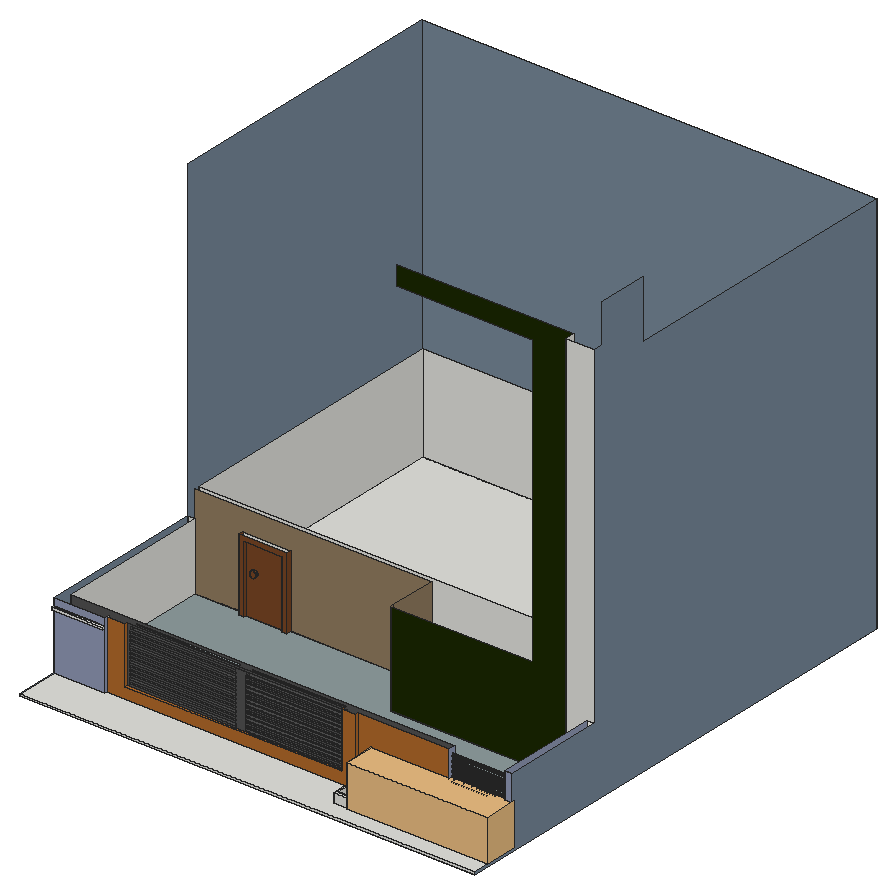
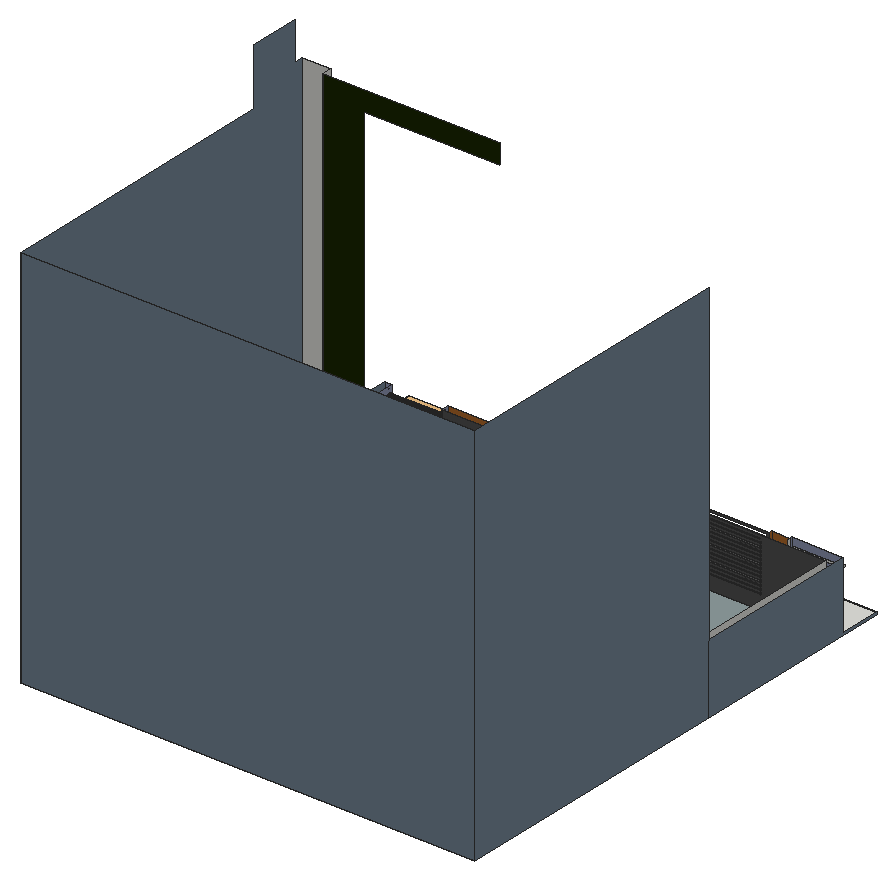
# SketchUp Ruby script. Lengths in inches.
U = 1.inch
M = Sketchup.active_model
def pt(a) = Geom::Point3d.new(a.map { |v| v * U })
def face(e, loops, mat)
  f = e.add_face(loops[0].map { |a| pt(a) })
  loops[1..].each { |l| e.add_face(l.map { |a| pt(a) }).erase! }
  f.material = f.back_material = mat if mat
  f
end
# faces: each face lists its corners as indices into pts; further lists are holes
def faces(e, pts, list, mat = nil) = list.each { |f| face(e, (f[0].is_a?(Array) ? f : [f]).map { |l| l.map { |i| pts[i] } }, mat) }
# xy, xz, yz: faces in a plane at the given z, y or x. An outline is a flat list of corners, or four numbers for a rectangle; further outlines are holes
def ring(l) = l.size == 4 ? [[l[0], l[1]], [l[2], l[1]], [l[2], l[3]], [l[0], l[3]]] : l.each_slice(2).to_a
def flat(e, list, mat, &to3) = list.each { |f| face(e, (f[0].is_a?(Array) ? f : [f]).map { |l| ring(l).map { |u, v| to3.(u, v) } }, mat) }
def xy(e, z, list, mat = nil) = flat(e, list, mat) { |x, y| [x, y, z] }
def xz(e, y, list, mat = nil) = flat(e, list, mat) { |x, z| [x, y, z] }
def yz(e, x, list, mat = nil) = flat(e, list, mat) { |y, z| [x, y, z] }
def lines(e, pts, list) = list.each { |a, b| e.add_line(pt(pts[a]), pt(pts[b])) }
# prism: a flat outline (further loops are holes) pulled along v
def prism(e, loops, v, mat = nil)
  f = face(e, loops, mat); d = Geom::Vector3d.new(v.map { |x| x * U })
  f.pushpull(f.normal.samedirection?(d) ? d.length : -d.length)
end
def box(e, o, s, mat = nil) = prism(e, [[o, [o[0] + s[0], o[1], o[2]], [o[0] + s[0], o[1] + s[1], o[2]], [o[0], o[1] + s[1], o[2]]]], [0, 0, s[2]], mat)
def at(x, y, z, deg = 0) = Geom::Transformation.translation(pt([x, y, z])) * Geom::Transformation.rotation(ORIGIN, Z_AXIS, deg.degrees)
def axes(o, x, y, z) = Geom::Transformation.new([*x, 0, *y, 0, *z, 0, *pt(o).to_a, 1])
def part(name) = M.definitions.add(name)
# library, detail: a bought-in or finely detailed component or shape, given as its bounding box
def library(name, o, s) = part(name).tap { |d| box(d.entities, o, s) }
def detail(e, o, s) = box(e.add_group.entities, o, s)
def put(e, d, t, mat = nil) = e.add_instance(d, t).tap { |i| i.material = mat if mat }
def group(e, t, mat = nil) = e.add_group.tap { |g| g.transformation = t; g.material = mat if mat }.entities
root = M.entities
M.materials.add("Niraj_Shirt").color = [144, 153, 181]
M.materials.add("[0035_Tan]").color = [145, 124, 96]
M.materials.add("[0060_GrassGreen]").color = [27, 40, 2]
M.materials.add("[0110_LightSlateGray]").color = [119, 136, 153]
M.materials.add("[0135_DarkGray]").color = [81, 81, 81]
M.materials.add("[0136_Charcoal]").color = [35, 35, 35]
M.materials.add("[Metal Panel]").color = [143, 157, 158]
M.materials.add("[Wood Bamboo]").color = [177, 105, 43]
M.materials.add("[Wood Veneer 01]").color = [120, 70, 37]
c1 = library("Potted flowering plants",[-0.05,-0.05,0],[59.02,14.54,22.0625])
xy(root,0,[[3.53,0,3.53,261.0625,307.22,261.0625,307.22,198.0625,534.65,198.0625,534.65,186.0625,569.78,186.0625,569.78,0],[534.65,186.0625,569.78,198.0625],[307.22,198.0625,450.59,261.0625],[450.59,198.0625,459.59,261.0625],[459.59,198.0625,569.78,261.0625],
  [[3.53,261.0625,569.78,625.1875],[12.53,267.0625,450.59,616.1875]],[12.53,267.0625,450.59,616.1875]])
xy(root,3,[[3.53,0,569.78,0,569.78,20.66,377.85,20.66,377.85,55.23,67.4,55.23,67.4,52.23,3.53,52.23],[381.12,23.93,566.51,58.23],[71.58,255.0625,77.58,261.0625],[125.58,255.0625,131.58,261.0625],[77.58,258.0625,125.58,261.0625]])
xy(root,3,[[12.53,67.23,560.78,67.23,560.78,186.0625,534.65,186.0625,534.65,198.0625,307.22,198.0625,307.22,261.0625,131.58,261.0625,131.58,255.0625,125.58,255.0625,125.58,258.0625,77.58,258.0625,77.58,255.0625,71.58,255.0625,71.58,261.0625,12.53,261.0625]],"[Metal Panel]")
xy(root,15,[[377.85,20.66,569.78,20.66,569.78,58.23,566.51,58.23,566.51,23.93,381.12,23.93,381.12,58.23,377.85,58.23]])
xy(root,17.19,[[90.07,55.23,224.96,58.23],[224.96,55.23,238.29,58.23],[238.29,55.23,359.85,58.23]],"[Wood Bamboo]")
xy(root,18.47,[[238.29,58.23,356.85,67.23]],"[0135_DarkGray]")
xy(root,19.75,[[93.07,58.23,224.96,67.23]],"[0135_DarkGray]")
xy(root,21.1875,[[238.29,58.23,356.85,67.23]],"[0135_DarkGray]")
xy(root,22.25,[[93.07,58.23,224.96,67.23]],"[0135_DarkGray]")
xy(root,22.66,[[238.29,58.23,356.85,67.23]],"[0135_DarkGray]")
xy(root,24.5,[[93.07,58.23,224.96,67.23]],"[0135_DarkGray]")
xy(root,25.375,[[238.29,58.23,356.85,67.23]],"[0135_DarkGray]")
xy(root,26.85,[[238.29,58.23,356.85,67.23]],"[0135_DarkGray]")
xy(root,27,[[93.07,58.23,224.96,67.23]],"[0135_DarkGray]")
xy(root,29.25,[[93.07,58.23,224.96,67.23]],"[0135_DarkGray]")
xy(root,29.5625,[[238.29,58.23,356.85,67.23]],"[0135_DarkGray]")
xy(root,31.03,[[238.29,58.23,356.85,67.23]],"[0135_DarkGray]")
xy(root,31.75,[[93.07,58.23,224.96,67.23]],"[0135_DarkGray]")
xy(root,33.75,[[238.29,58.23,356.85,67.23]],"[0135_DarkGray]")
xy(root,34,[[93.07,58.23,224.96,67.23]],"[0135_DarkGray]")
xy(root,35.22,[[238.29,58.23,356.85,67.23]],"[0135_DarkGray]")
xy(root,36.5,[[93.07,58.23,224.96,67.23]],"[0135_DarkGray]")
xy(root,37.9375,[[238.29,58.23,356.85,67.23]],"[0135_DarkGray]")
xy(root,38.75,[[93.07,58.23,224.96,67.23]],"[0135_DarkGray]")
xy(root,39.41,[[238.29,58.23,356.85,67.23]],"[0135_DarkGray]")
xy(root,41.25,[[93.07,58.23,224.96,67.23]],"[0135_DarkGray]")
xy(root,42.125,[[238.29,58.23,356.85,67.23]],"[0135_DarkGray]")
xy(root,43.5,[[93.07,58.23,224.96,67.23]],"[0135_DarkGray]")
xy(root,43.6,[[238.29,58.23,356.85,67.23]],"[0135_DarkGray]")
xy(root,45,[[491.3125,58.23,560.78,67.23]],"Niraj_Shirt")
xy(root,46,[[93.07,58.23,224.96,67.23]],"[0135_DarkGray]")
xy(root,46.3125,[[238.29,58.23,356.85,67.23]],"[0135_DarkGray]")
xy(root,47.78,[[238.29,58.23,356.85,67.23]],"[0135_DarkGray]")
xy(root,48.25,[[93.07,58.23,224.96,67.23]],"[0135_DarkGray]")
xy(root,50.5,[[238.29,58.23,356.85,67.23]],"[0135_DarkGray]")
xy(root,50.75,[[93.07,58.23,224.96,67.23]],"[0135_DarkGray]")
xy(root,51.97,[[238.29,58.23,356.85,67.23]],"[0135_DarkGray]")
xy(root,53,[[93.07,58.23,224.96,67.23]],"[0135_DarkGray]")
xy(root,54.6875,[[238.29,58.23,356.85,67.23]],"[0135_DarkGray]")
xy(root,55.5,[[93.07,58.23,224.96,67.23]],"[0135_DarkGray]")
xy(root,56.16,[[238.29,58.23,356.85,67.23]],"[0135_DarkGray]")
xy(root,57.75,[[93.07,58.23,224.96,67.23]],"[0135_DarkGray]")
xy(root,58.875,[[238.29,58.23,356.85,67.23]],"[0135_DarkGray]")
xy(root,60.25,[[93.07,58.23,224.96,67.23]],"[0135_DarkGray]")
xy(root,60.35,[[238.29,58.23,356.85,67.23]],"[0135_DarkGray]")
xy(root,62.5,[[93.07,58.23,224.96,67.23]],"[0135_DarkGray]")
xy(root,63.0625,[[238.29,58.23,356.85,67.23]],"[0135_DarkGray]")
xy(root,64.53,[[238.29,58.23,356.85,67.23]],"[0135_DarkGray]")
xy(root,65,[[93.07,58.23,224.96,67.23]],"[0135_DarkGray]")
xy(root,67.25,[[93.07,58.23,224.96,67.23],[238.29,58.23,356.85,67.23]],"[0135_DarkGray]")
xy(root,68.72,[[238.29,58.23,356.85,67.23]],"[0135_DarkGray]")
xy(root,69.75,[[93.07,58.23,224.96,67.23]],"[0135_DarkGray]")
xy(root,71.4375,[[238.29,58.23,356.85,67.23]],"[0135_DarkGray]")
xy(root,72,[[93.07,58.23,224.96,67.23]],"[0135_DarkGray]")
xy(root,72.91,[[238.29,58.23,356.85,67.23]],"[0135_DarkGray]")
xy(root,74.5,[[93.07,58.23,224.96,67.23]],"[0135_DarkGray]")
xy(root,74.66,[[3.53,49.23,67.4,52.23]])
xy(root,75.625,[[238.29,58.23,356.85,67.23]],"[0135_DarkGray]")
xy(root,76.75,[[93.07,58.23,224.96,67.23]],"[0135_DarkGray]")
xy(root,77.1,[[238.29,58.23,356.85,67.23]],"[0135_DarkGray]")
xy(root,77.67,[[3.53,49.23,67.4,52.23]])
xy(root,79.25,[[93.07,58.23,224.96,67.23]],"[0135_DarkGray]")
xy(root,79.8125,[[238.29,58.23,356.85,67.23]],"[0135_DarkGray]")
xz(root,0,[[3.53,0,569.78,3]])
xz(root,20.66,[[377.85,3,569.78,15]])
xz(root,23.93,[[381.12,3,566.51,15]])
xz(root,49.23,[[3.53,74.66,67.4,77.67]])
xz(root,52.23,[[3.53,74.66,67.4,77.67]])
xz(root,52.23,[[3.53,3,67.4,74.66],[3.53,77.67,67.4,87]],"Niraj_Shirt")
xz(root,55.23,[[67.4,3,377.85,3,377.85,87,359.85,87,359.85,17.19,90.07,17.19,90.07,87,67.4,87]],"[Wood Bamboo]")
xz(root,58.23,[[377.85,3,381.12,15]])
xz(root,58.23,[[491.09,3,566.51,3,566.51,15,569.78,15,569.78,87,560.78,87,560.78,45,491.3125,45,491.3125,87,491.09,87]],"Niraj_Shirt")
xz(root,58.23,[[90.07,17.19,224.96,17.19,224.96,19.75,93.07,19.75,93.07,84,356.85,84,356.85,18.47,238.29,18.47,238.29,17.19,359.85,17.19,359.85,87,90.07,87],[224.96,17.19,238.29,84],[238.29,21.1875,356.85,22.66],[93.07,22.25,224.96,24.5],[238.29,25.375,356.85,26.85],
  [93.07,27,224.96,29.25],[238.29,29.5625,356.85,31.03],[93.07,31.75,224.96,34],[238.29,33.75,356.85,35.22],[93.07,36.5,224.96,38.75],
  [238.29,37.9375,356.85,39.41],[93.07,41.25,224.96,43.5],[238.29,42.125,356.85,43.6],[93.07,46,224.96,48.25],[238.29,46.3125,356.85,47.78],
  [238.29,50.5,356.85,51.97],[93.07,50.75,224.96,53],[238.29,54.6875,356.85,56.16],[93.07,55.5,224.96,57.75],[238.29,58.875,356.85,60.35],
  [93.07,60.25,224.96,62.5],[238.29,63.0625,356.85,64.53],[93.07,65,224.96,67.25],[238.29,67.25,356.85,68.72],[93.07,69.75,224.96,72],
  [238.29,71.4375,356.85,72.91],[93.07,74.5,224.96,76.75],[238.29,75.625,356.85,77.1],[93.07,79.25,224.96,81.5],[238.29,79.8125,356.85,81.28]],"[0135_DarkGray]")
xz(root,58.23,[[381.12,3,491.09,3,491.09,87,377.85,87,377.85,15,381.12,15]],"[Wood Bamboo]")
xz(root,67.23,[[[12.53,3,12.53,87,491.3125,87,491.3125,45,560.78,45,560.78,3],[93.07,81.5,224.96,84],[93.07,76.75,224.96,79.25],[93.07,72,224.96,74.5],[93.07,67.25,224.96,69.75],[93.07,62.5,224.96,65],[93.07,57.75,224.96,60.25],[93.07,53,224.96,55.5],[93.07,48.25,224.96,50.75],[93.07,43.5,224.96,46],[93.07,38.75,224.96,41.25],[93.07,34,224.96,36.5],[93.07,29.25,224.96,31.75],[93.07,24.5,224.96,27],[93.07,19.75,224.96,22.25],[238.29,18.47,356.85,21.1875],[238.29,81.28,356.85,84],[238.29,77.1,356.85,79.8125],[238.29,72.91,356.85,75.625],[238.29,68.72,356.85,71.4375],[238.29,64.53,356.85,67.25],[238.29,60.35,356.85,63.0625],[238.29,56.16,356.85,58.875],[238.29,51.97,356.85,54.6875],[238.29,47.78,356.85,50.5],[238.29,43.6,356.85,46.3125],[238.29,39.41,356.85,42.125],[238.29,35.22,356.85,37.9375],[238.29,31.03,356.85,33.75],[238.29,26.85,356.85,29.5625],[238.29,22.66,356.85,25.375]]],"[0135_DarkGray]")
xz(root,186.0625,[[534.65,3,560.78,3,560.78,87,569.78,87,569.78,504.07,534.65,504.07]])
xz(root,198.0625,[[307.22,0,450.59,3],[450.59,0,534.65,3]])
xz(root,198.0625,[[307.22,3,534.65,3,534.65,504.07,314.59,504.07,314.59,480,483.9,480,483.9,120,307.22,120]],"[0060_GrassGreen]")
xz(root,255.0625,[[71.58,3,77.58,3,77.58,87,125.58,87,125.58,3,131.58,3,131.58,93,71.58,93],[88.84,49.68,89.86,49.82,90.8125,50.21,91.63,50.84,92.25,51.65,92.65,52.6,92.78,53.62,92.65,54.64,92.25,55.59,91.63,56.41,90.8125,57.03,89.86,57.42,88.84,57.56,87.83,57.42,86.875,57.03,86.0625,56.41,85.43,55.59,85.04,54.64,84.91,53.62,85.04,52.6,85.43,51.65,86.0625,50.84,86.875,50.21,87.83,49.82]],"[Wood Veneer 01]")
xz(root,258.0625,[[88.84,49.68,87.83,49.82,86.875,50.21,86.0625,50.84,85.43,51.65,85.04,52.6,84.91,53.62,85.04,54.64,85.43,55.59,86.0625,56.41,86.875,57.03,87.83,57.42,88.84,57.56,89.86,57.42,90.8125,57.03,91.63,56.41,92.25,55.59,92.65,54.64,92.78,53.62,92.65,52.6,92.25,51.65,91.63,50.84,90.8125,50.21,89.86,49.82]])
xz(root,258.0625,[[[77.58,3,125.58,87],[88.84,49.68,87.83,49.82,86.875,50.21,86.0625,50.84,85.43,51.65,85.04,52.6,84.91,53.62,85.04,54.64,85.43,55.59,86.0625,56.41,86.875,57.03,87.83,57.42,88.84,57.56,89.86,57.42,90.8125,57.03,91.63,56.41,92.25,55.59,92.65,54.64,92.78,53.62,92.65,52.6,92.25,51.65,91.63,50.84,90.8125,50.21,89.86,49.82]]],"[Wood Veneer 01]")
xz(root,261.0625,[[3.53,0,12.53,3],[12.53,0,71.58,3],[71.58,0,131.58,3],[131.58,0,307.22,3],[3.53,3,12.53,87]])
xz(root,261.0625,[[12.53,3,71.58,3,71.58,93,131.58,93,131.58,3,307.22,3,307.22,120,12.53,120]],"[0035_Tan]")
xz(root,267.0625,[[12.53,0,450.59,120]])
xz(root,616.1875,[[12.53,0,450.59,120]])
xz(root,625.1875,[[3.53,0,569.78,480]],"[0110_LightSlateGray]")
yz(root,3.53,[[49.23,74.66,52.23,77.67]])
yz(root,3.53,[[0,0,0,3,52.23,3,52.23,87,261.0625,87,261.0625,0],[261.0625,0,625.1875,480]],"[0110_LightSlateGray]")
yz(root,12.53,[[267.0625,0,616.1875,120],[67.23,3,261.0625,87]])
yz(root,67.4,[[55.23,3,58.23,87],[49.23,74.66,52.23,77.67]])
yz(root,67.4,[[52.23,3,55.23,87]],"Niraj_Shirt")
yz(root,71.58,[[255.0625,3,261.0625,93]],"[Wood Veneer 01]")
yz(root,77.58,[[255.0625,3,258.0625,87]],"[Wood Veneer 01]")
yz(root,90.07,[[55.23,17.19,58.23,87]],"[Wood Bamboo]")
yz(root,93.07,[[58.23,19.75,67.23,22.25],[58.23,24.5,67.23,27],[58.23,29.25,67.23,31.75],[58.23,34,67.23,36.5],[58.23,38.75,67.23,41.25],
  [58.23,43.5,67.23,46],[58.23,48.25,67.23,50.75],[58.23,53,67.23,55.5],[58.23,57.75,67.23,60.25],[58.23,62.5,67.23,65],
  [58.23,67.25,67.23,69.75],[58.23,72,67.23,74.5],[58.23,76.75,67.23,79.25]],"[0135_DarkGray]")
yz(root,125.58,[[255.0625,3,258.0625,87]],"[Wood Veneer 01]")
yz(root,131.58,[[255.0625,3,261.0625,93]],"[Wood Veneer 01]")
yz(root,224.96,[[58.23,19.75,67.23,22.25],[58.23,24.5,67.23,27],[58.23,29.25,67.23,31.75],[58.23,34,67.23,36.5],[58.23,38.75,67.23,41.25],
  [58.23,43.5,67.23,46],[58.23,48.25,67.23,50.75],[58.23,53,67.23,55.5],[58.23,57.75,67.23,60.25],[58.23,62.5,67.23,65],
  [58.23,67.25,67.23,69.75],[58.23,72,67.23,74.5],[58.23,76.75,67.23,79.25]],"[0135_DarkGray]")
yz(root,238.29,[[58.23,18.47,67.23,20.19],[58.23,20.19,67.23,21.1875],[58.23,22.66,67.23,25.375],[58.23,26.85,67.23,29.5625],[58.23,31.03,67.23,33.75],
  [58.23,35.22,67.23,37.9375],[58.23,39.41,67.23,42.125],[58.23,43.6,67.23,46.3125],[58.23,47.78,67.23,50.5],[58.23,51.97,67.23,54.6875],
  [58.23,56.16,67.23,58.875],[58.23,60.35,67.23,63.0625],[58.23,64.53,67.23,67.25],[58.23,68.72,67.23,71.4375],[58.23,72.91,67.23,75.625],
  [58.23,77.1,67.23,79.8125]],"[0135_DarkGray]")
yz(root,307.22,[[198.0625,0,201.0625,3],[201.0625,0,261.0625,3]])
yz(root,307.22,[[198.0625,3,201.0625,120],[201.0625,3,261.0625,120]],"[0035_Tan]")
yz(root,356.85,[[58.23,18.47,67.23,20.19],[58.23,20.19,67.23,21.1875],[58.23,22.66,67.23,25.375],[58.23,26.85,67.23,29.5625],[58.23,31.03,67.23,33.75],
  [58.23,35.22,67.23,37.9375],[58.23,39.41,67.23,42.125],[58.23,43.6,67.23,46.3125],[58.23,47.78,67.23,50.5],[58.23,51.97,67.23,54.6875],
  [58.23,56.16,67.23,58.875],[58.23,60.35,67.23,63.0625],[58.23,64.53,67.23,67.25],[58.23,68.72,67.23,71.4375],[58.23,72.91,67.23,75.625],
  [58.23,77.1,67.23,79.8125]],"[0135_DarkGray]")
yz(root,359.85,[[55.23,17.19,58.23,87]],"[Wood Bamboo]")
yz(root,377.85,[[20.66,3,55.23,15]])
yz(root,377.85,[[55.23,15,58.23,87]],"[Wood Bamboo]")
yz(root,381.12,[[23.93,3,58.23,15]])
yz(root,450.59,[[267.0625,0,616.1875,120]])
yz(root,491.3125,[[62.8,41.92,63.2,41.97,63.58,42.125,63.91,42.375,64.15,42.7,64.31,43.07,64.36,43.48,64.31,43.88,64.15,44.26,63.91,44.58,63.58,44.83,63.2,44.99,63.12,45,62.48,45,62.4,44.99,62.02,44.83,61.7,44.58,61.45,44.26,61.29,43.88,61.24,43.48,61.29,43.07,61.45,42.7,61.7,42.375,62.02,42.125,62.4,41.97],[62.48,45,63.12,45,62.8,45.04]])
yz(root,491.3125,[[[58.23,45,62.48,45,62.8,45.04,63.12,45,67.23,45,67.23,87,58.23,87],[62.8,82.6,62.4,82.66,62.02,82.8125,61.7,83.0625,61.45,83.39,61.29,83.76,61.24,84.17,61.29,84.57,61.45,84.95,61.7,85.27,62.02,85.52,62.4,85.68,62.8,85.73,63.2,85.68,63.58,85.52,63.91,85.27,64.15,84.95,64.31,84.57,64.36,84.17,64.31,83.76,64.15,83.39,63.91,83.0625,63.58,82.8125,63.2,82.66],[62.8,76.79,62.4,76.85,62.02,77,61.7,77.25,61.45,77.57,61.29,77.95,61.24,78.35,61.29,78.76,61.45,79.14,61.7,79.46,62.02,79.71,62.4,79.86,62.8,79.92,63.2,79.86,63.58,79.71,63.91,79.46,64.15,79.14,64.31,78.76,64.36,78.35,64.31,77.95,64.15,77.57,63.91,77.25,63.58,77,63.2,76.85],[62.8,70.98,62.4,71.03,62.02,71.1875,61.7,71.4375,61.45,71.76,61.29,72.14,61.24,72.54,61.29,72.95,61.45,73.32,61.7,73.65,62.02,73.9,62.4,74.05,62.8,74.1,63.2,74.05,63.58,73.9,63.91,73.65,64.15,73.32,64.31,72.95,64.36,72.54,64.31,72.14,64.15,71.76,63.91,71.4375,63.58,71.1875,63.2,71.03],[62.8,65.17,62.4,65.22,62.02,65.375,61.7,65.625,61.45,65.95,61.29,66.32,61.24,66.73,61.29,67.13,61.45,67.51,61.7,67.83,62.02,68.08,62.4,68.24,62.8,68.29,63.2,68.24,63.58,68.08,63.91,67.83,64.15,67.51,64.31,67.13,64.36,66.73,64.31,66.32,64.15,65.95,63.91,65.625,63.58,65.375,63.2,65.22],[62.8,59.35,62.4,59.41,62.02,59.5625,61.7,59.8125,61.45,60.14,61.29,60.51,61.24,60.92,61.29,61.32,61.45,61.7,61.7,62.02,62.02,62.27,62.4,62.43,62.8,62.48,63.2,62.43,63.58,62.27,63.91,62.02,64.15,61.7,64.31,61.32,64.36,60.92,64.31,60.51,64.15,60.14,63.91,59.8125,63.58,59.5625,63.2,59.41],[62.8,53.54,62.4,53.6,62.02,53.75,61.7,54,61.45,54.32,61.29,54.7,61.24,55.1,61.29,55.51,61.45,55.89,61.7,56.21,62.02,56.46,62.4,56.61,62.8,56.67,63.2,56.61,63.58,56.46,63.91,56.21,64.15,55.89,64.31,55.51,64.36,55.1,64.31,54.7,64.15,54.32,63.91,54,63.58,53.75,63.2,53.6],[62.8,47.73,62.4,47.78,62.02,47.9375,61.7,48.1875,61.45,48.51,61.29,48.89,61.24,49.29,61.29,49.7,61.45,50.07,61.7,50.4,62.02,50.65,62.4,50.8,62.8,50.85,63.2,50.8,63.58,50.65,63.91,50.4,64.15,50.07,64.31,49.7,64.36,49.29,64.31,48.89,64.15,48.51,63.91,48.1875,63.58,47.9375,63.2,47.78]]],"Niraj_Shirt")
yz(root,534.65,[[186.0625,0,198.0625,3],[186.0625,3,198.0625,504.07]])
yz(root,560.4375,[[62.8,47.73,63.2,47.78,63.58,47.9375,63.91,48.1875,64.15,48.51,64.31,48.89,64.36,49.29,64.31,49.7,64.15,50.07,63.91,50.4,63.58,50.65,63.2,50.8,62.8,50.85,62.4,50.8,62.02,50.65,61.7,50.4,61.45,50.07,61.29,49.7,61.24,49.29,61.29,48.89,61.45,48.51,61.7,48.1875,62.02,47.9375,62.4,47.78]])
yz(root,560.78,[[[67.23,3,67.23,45,58.23,45,58.23,87,186.0625,87,186.0625,3],[62.8,82.6,63.2,82.66,63.58,82.8125,63.91,83.0625,64.15,83.39,64.31,83.76,64.36,84.17,64.31,84.57,64.15,84.95,63.91,85.27,63.58,85.52,63.2,85.68,62.8,85.73,62.4,85.68,62.02,85.52,61.7,85.27,61.45,84.95,61.29,84.57,61.24,84.17,61.29,83.76,61.45,83.39,61.7,83.0625,62.02,82.8125,62.4,82.66],[62.8,76.79,63.2,76.85,63.58,77,63.91,77.25,64.15,77.57,64.31,77.95,64.36,78.35,64.31,78.76,64.15,79.14,63.91,79.46,63.58,79.71,63.2,79.86,62.8,79.92,62.4,79.86,62.02,79.71,61.7,79.46,61.45,79.14,61.29,78.76,61.24,78.35,61.29,77.95,61.45,77.57,61.7,77.25,62.02,77,62.4,76.85],[62.8,70.98,63.2,71.03,63.58,71.1875,63.91,71.4375,64.15,71.76,64.31,72.14,64.36,72.54,64.31,72.95,64.15,73.32,63.91,73.65,63.58,73.9,63.2,74.05,62.8,74.1,62.4,74.05,62.02,73.9,61.7,73.65,61.45,73.32,61.29,72.95,61.24,72.54,61.29,72.14,61.45,71.76,61.7,71.4375,62.02,71.1875,62.4,71.03]]],"Niraj_Shirt")
yz(root,562.0625,[[62.8,59.35,63.2,59.41,63.58,59.5625,63.91,59.8125,64.15,60.14,64.31,60.51,64.36,60.92,64.31,61.32,64.15,61.7,63.91,62.02,63.58,62.27,63.2,62.43,62.8,62.48,62.4,62.43,62.02,62.27,61.7,62.02,61.45,61.7,61.29,61.32,61.24,60.92,61.29,60.51,61.45,60.14,61.7,59.8125,62.02,59.5625,62.4,59.41]])
yz(root,562.125,[[62.8,65.17,63.2,65.22,63.58,65.375,63.91,65.625,64.15,65.95,64.31,66.32,64.36,66.73,64.31,67.13,64.15,67.51,63.91,67.83,63.58,68.08,63.2,68.24,62.8,68.29,62.4,68.24,62.02,68.08,61.7,67.83,61.45,67.51,61.29,67.13,61.24,66.73,61.29,66.32,61.45,65.95,61.7,65.625,62.02,65.375,62.4,65.22]])
yz(root,562.4375,[[62.8,53.54,63.2,53.6,63.58,53.75,63.91,54,64.15,54.32,64.31,54.7,64.36,55.1,64.31,55.51,64.15,55.89,63.91,56.21,63.58,56.46,63.2,56.61,62.8,56.67,62.4,56.61,62.02,56.46,61.7,56.21,61.45,55.89,61.29,55.51,61.24,55.1,61.29,54.7,61.45,54.32,61.7,54,62.02,53.75,62.4,53.6]])
yz(root,566.51,[[23.93,3,58.23,15]])
yz(root,569.78,[[0,0,625.1875,0,625.1875,480,261.0625,480,261.0625,551.875,198.0625,551.875,198.0625,504.07,186.0625,504.07,186.0625,87,58.23,87,58.23,15,20.66,15,20.66,3,0,3]],"[0110_LightSlateGray]")
p = [[491.3125,62.4,47.78],[491.3125,62.8,47.73],[560.4375,62.8,47.73],[560.4375,62.4,47.78],[491.3125,63.2,47.78],[560.4375,63.2,47.78],
  [491.3125,62.02,47.9375],[560.4375,62.02,47.9375],[491.3125,63.58,47.9375],[560.4375,63.58,47.9375],[491.3125,61.7,48.1875],[560.4375,61.7,48.1875],
  [491.3125,63.91,48.1875],[560.4375,63.91,48.1875],[491.3125,61.45,48.51],[560.4375,61.45,48.51],[491.3125,64.15,48.51],[560.4375,64.15,48.51],
  [491.3125,61.29,48.89],[560.4375,61.29,48.89],[491.3125,64.31,48.89],[560.4375,64.31,48.89],[491.3125,61.24,49.29],[560.4375,61.24,49.29],
  [491.3125,64.36,49.29],[560.4375,64.36,49.29],[491.3125,61.29,49.7],[560.4375,61.29,49.7],[491.3125,64.31,49.7],[560.4375,64.31,49.7],
  [491.3125,61.45,50.07],[560.4375,61.45,50.07],[491.3125,64.15,50.07],[560.4375,64.15,50.07],[87.83,258.0625,49.82],[88.84,258.0625,49.68],
  [88.84,255.0625,49.68],[87.83,255.0625,49.82],[89.86,258.0625,49.82],[89.86,255.0625,49.82],[86.875,258.0625,50.21],[86.875,255.0625,50.21],
  [90.8125,258.0625,50.21],[90.8125,255.0625,50.21],[491.3125,61.7,50.4],[560.4375,61.7,50.4],[491.3125,63.91,50.4],[560.4375,63.91,50.4],
  [86.0625,258.0625,50.84],[86.0625,255.0625,50.84],[91.63,258.0625,50.84],[91.63,255.0625,50.84],[491.3125,62.02,50.65],[560.4375,62.02,50.65],
  [491.3125,63.58,50.65],[560.4375,63.58,50.65],[491.3125,62.4,50.8],[560.4375,62.4,50.8],[491.3125,63.2,50.8],[560.4375,63.2,50.8],
  [491.3125,62.8,50.85],[560.4375,62.8,50.85],[85.43,258.0625,51.65],[85.43,255.0625,51.65],[92.25,258.0625,51.65],[92.25,255.0625,51.65],
  [85.04,258.0625,52.6],[85.04,255.0625,52.6],[92.65,258.0625,52.6],[92.65,255.0625,52.6],[84.91,258.0625,53.62],[84.91,255.0625,53.62],
  [92.78,258.0625,53.62],[92.78,255.0625,53.62],[491.3125,62.4,53.6],[491.3125,62.8,53.54],[562.4375,62.8,53.54],[562.4375,62.4,53.6],
  [491.3125,63.2,53.6],[562.4375,63.2,53.6],[491.3125,62.02,53.75],[562.4375,62.02,53.75],[491.3125,63.58,53.75],[562.4375,63.58,53.75],
  [85.04,258.0625,54.64],[85.04,255.0625,54.64],[92.65,258.0625,54.64],[92.65,255.0625,54.64],[491.3125,61.7,54],[562.4375,61.7,54],
  [491.3125,63.91,54],[562.4375,63.91,54],[491.3125,61.45,54.32],[562.4375,61.45,54.32],[491.3125,64.15,54.32],[562.4375,64.15,54.32],
  [491.3125,61.29,54.7],[562.4375,61.29,54.7],[491.3125,64.31,54.7],[562.4375,64.31,54.7],[85.43,258.0625,55.59],[85.43,255.0625,55.59],
  [92.25,258.0625,55.59],[92.25,255.0625,55.59],[491.3125,61.24,55.1],[562.4375,61.24,55.1],[491.3125,64.36,55.1],[562.4375,64.36,55.1],
  [491.3125,61.29,55.51],[562.4375,61.29,55.51],[491.3125,64.31,55.51],[562.4375,64.31,55.51],[491.3125,61.45,55.89],[562.4375,61.45,55.89],
  [491.3125,64.15,55.89],[562.4375,64.15,55.89],[86.0625,258.0625,56.41],[86.0625,255.0625,56.41],[91.63,258.0625,56.41],[91.63,255.0625,56.41],
  [491.3125,61.7,56.21],[562.4375,61.7,56.21],[491.3125,63.91,56.21],[562.4375,63.91,56.21],[491.3125,62.02,56.46],[562.4375,62.02,56.46],
  [491.3125,63.58,56.46],[562.4375,63.58,56.46],[86.875,258.0625,57.03],[86.875,255.0625,57.03],[90.8125,258.0625,57.03],[90.8125,255.0625,57.03],
  [491.3125,62.4,56.61],[562.4375,62.4,56.61],[491.3125,63.2,56.61],[562.4375,63.2,56.61],[491.3125,62.8,56.67],[562.4375,62.8,56.67],
  [87.83,258.0625,57.42],[87.83,255.0625,57.42],[89.86,258.0625,57.42],[89.86,255.0625,57.42],[88.84,258.0625,57.56],[88.84,255.0625,57.56],
  [491.3125,62.02,59.5625],[491.3125,62.4,59.41],[562.0625,62.4,59.41],[562.0625,62.02,59.5625],[491.3125,62.8,59.35],[562.0625,62.8,59.35],
  [491.3125,63.2,59.41],[562.0625,63.2,59.41],[491.3125,63.58,59.5625],[562.0625,63.58,59.5625],[491.3125,61.7,59.8125],[562.0625,61.7,59.8125],
  [491.3125,63.91,59.8125],[562.0625,63.91,59.8125],[491.3125,61.45,60.14],[562.0625,61.45,60.14],[491.3125,64.15,60.14],[562.0625,64.15,60.14],
  [491.3125,61.29,60.51],[562.0625,61.29,60.51],[491.3125,64.31,60.51],[562.0625,64.31,60.51],[491.3125,61.24,60.92],[562.0625,61.24,60.92],
  [491.3125,64.36,60.92],[562.0625,64.36,60.92],[491.3125,61.29,61.32],[562.0625,61.29,61.32],[491.3125,64.31,61.32],[562.0625,64.31,61.32],
  [491.3125,61.45,61.7],[562.0625,61.45,61.7],[491.3125,64.15,61.7],[562.0625,64.15,61.7],[491.3125,61.7,62.02],[562.0625,61.7,62.02],
  [491.3125,63.91,62.02],[562.0625,63.91,62.02],[491.3125,62.02,62.27],[562.0625,62.02,62.27],[491.3125,63.58,62.27],[562.0625,63.58,62.27],
  [491.3125,62.4,62.43],[562.0625,62.4,62.43],[491.3125,63.2,62.43],[562.0625,63.2,62.43],[491.3125,62.8,62.48],[562.0625,62.8,62.48],
  [491.3125,62.02,65.375],[491.3125,62.4,65.22],[562.125,62.4,65.22],[562.125,62.02,65.375],[491.3125,62.8,65.17],[562.125,62.8,65.17],
  [491.3125,63.2,65.22],[562.125,63.2,65.22],[491.3125,63.58,65.375],[562.125,63.58,65.375],[491.3125,61.7,65.625],[562.125,61.7,65.625],
  [491.3125,63.91,65.625],[562.125,63.91,65.625],[491.3125,61.45,65.95],[562.125,61.45,65.95],[491.3125,64.15,65.95],[562.125,64.15,65.95],
  [491.3125,61.29,66.32],[562.125,61.29,66.32],[491.3125,64.31,66.32],[562.125,64.31,66.32],[491.3125,61.24,66.73],[562.125,61.24,66.73],
  [491.3125,64.36,66.73],[562.125,64.36,66.73],[491.3125,61.29,67.13],[562.125,61.29,67.13],[491.3125,64.31,67.13],[562.125,64.31,67.13],
  [491.3125,61.45,67.51],[562.125,61.45,67.51],[491.3125,64.15,67.51],[562.125,64.15,67.51],[491.3125,61.7,67.83],[562.125,61.7,67.83],
  [491.3125,63.91,67.83],[562.125,63.91,67.83],[491.3125,62.02,68.08],[562.125,62.02,68.08],[491.3125,63.58,68.08],[562.125,63.58,68.08],
  [491.3125,62.4,68.24],[562.125,62.4,68.24],[491.3125,63.2,68.24],[562.125,63.2,68.24],[491.3125,62.8,68.29],[562.125,62.8,68.29],
  [491.3125,62.02,71.1875],[491.3125,62.4,71.03],[560.78,62.4,71.03],[560.78,62.02,71.1875],[491.3125,62.8,70.98],[560.78,62.8,70.98],
  [491.3125,63.2,71.03],[560.78,63.2,71.03],[491.3125,63.58,71.1875],[560.78,63.58,71.1875],[491.3125,61.7,71.4375],[560.78,61.7,71.4375],
  [491.3125,63.91,71.4375],[560.78,63.91,71.4375],[491.3125,61.45,71.76],[560.78,61.45,71.76],[491.3125,64.15,71.76],[560.78,64.15,71.76],
  [491.3125,61.29,72.14],[560.78,61.29,72.14],[491.3125,64.31,72.14],[560.78,64.31,72.14],[491.3125,61.24,72.54],[560.78,61.24,72.54],
  [491.3125,64.36,72.54],[560.78,64.36,72.54],[491.3125,61.29,72.95],[560.78,61.29,72.95],[491.3125,64.31,72.95],[560.78,64.31,72.95],
  [491.3125,61.45,73.32],[560.78,61.45,73.32],[491.3125,64.15,73.32],[560.78,64.15,73.32],[491.3125,61.7,73.65],[560.78,61.7,73.65],
  [491.3125,63.91,73.65],[560.78,63.91,73.65],[491.3125,62.02,73.9],[560.78,62.02,73.9],[491.3125,63.58,73.9],[560.78,63.58,73.9],
  [491.3125,62.4,74.05],[560.78,62.4,74.05],[491.3125,63.2,74.05],[560.78,63.2,74.05],[491.3125,62.8,74.1],[560.78,62.8,74.1],
  [491.3125,62.02,77],[491.3125,62.4,76.85],[560.78,62.4,76.85],[560.78,62.02,77],[491.3125,62.8,76.79],[560.78,62.8,76.79],
  [491.3125,63.2,76.85],[560.78,63.2,76.85],[491.3125,63.58,77],[560.78,63.58,77],[491.3125,61.7,77.25],[560.78,61.7,77.25],
  [491.3125,63.91,77.25],[560.78,63.91,77.25],[491.3125,61.45,77.57],[560.78,61.45,77.57],[491.3125,64.15,77.57],[560.78,64.15,77.57],
  [491.3125,61.29,77.95],[560.78,61.29,77.95],[491.3125,64.31,77.95],[560.78,64.31,77.95],[491.3125,61.24,78.35],[560.78,61.24,78.35],
  [491.3125,64.36,78.35],[560.78,64.36,78.35],[491.3125,61.29,78.76],[560.78,61.29,78.76],[491.3125,64.31,78.76],[560.78,64.31,78.76],
  [491.3125,61.45,79.14],[560.78,61.45,79.14],[491.3125,64.15,79.14],[560.78,64.15,79.14],[491.3125,61.7,79.46],[560.78,61.7,79.46],
  [491.3125,63.91,79.46],[560.78,63.91,79.46],[491.3125,62.02,79.71],[560.78,62.02,79.71],[491.3125,63.58,79.71],[560.78,63.58,79.71],
  [491.3125,62.4,79.86],[560.78,62.4,79.86],[491.3125,63.2,79.86],[560.78,63.2,79.86],[491.3125,62.8,79.92],[560.78,62.8,79.92],
  [3.53,58.23,3],[67.4,58.23,3]]
faces(root,p,[[0,1,2,3],[1,4,5,2],[6,0,3,7],[4,8,9,5],[10,6,7,11],[8,12,13,9],[14,10,11,15],[12,16,17,13],
  [18,14,15,19],[16,20,21,17],[22,18,19,23],[20,24,25,21],[26,22,23,27],[24,28,29,25],[30,26,27,31],[28,32,33,29],
  [44,30,31,45],[32,46,47,33],[52,44,45,53],[46,54,55,47],[56,52,53,57],[54,58,59,55],[60,56,57,61],[58,60,61,59],
  [74,75,76,77],[75,78,79,76],[80,74,77,81],[78,82,83,79],[88,80,81,89],[82,90,91,83],[92,88,89,93],[90,94,95,91],
  [96,92,93,97],[94,98,99,95],[104,96,97,105],[98,106,107,99],[108,104,105,109],[106,110,111,107],[112,108,109,113],[110,114,115,111],
  [120,112,113,121],[114,122,123,115],[124,120,121,125],[122,126,127,123],[132,124,125,133],[126,134,135,127],[136,132,133,137],[134,136,137,135],
  [144,145,146,147],[145,148,149,146],[148,150,151,149],[150,152,153,151],[154,144,147,155],[152,156,157,153],[158,154,155,159],[156,160,161,157],
  [162,158,159,163],[160,164,165,161],[166,162,163,167],[164,168,169,165],[170,166,167,171],[168,172,173,169],[174,170,171,175],[172,176,177,173],
  [178,174,175,179],[176,180,181,177],[182,178,179,183],[180,184,185,181],[186,182,183,187],[184,188,189,185],[190,186,187,191],[188,190,191,189],
  [192,193,194,195],[193,196,197,194],[196,198,199,197],[198,200,201,199],[202,192,195,203],[200,204,205,201],[206,202,203,207],[204,208,209,205],
  [210,206,207,211],[208,212,213,209],[214,210,211,215],[212,216,217,213],[218,214,215,219],[216,220,221,217],[222,218,219,223],[220,224,225,221],
  [226,222,223,227],[224,228,229,225],[230,226,227,231],[228,232,233,229],[234,230,231,235],[232,236,237,233],[238,234,235,239],[236,238,239,237],
  [240,241,242,243],[241,244,245,242],[244,246,247,245],[246,248,249,247],[250,240,243,251],[248,252,253,249],[254,250,251,255],[252,256,257,253],
  [258,254,255,259],[256,260,261,257],[262,258,259,263],[260,264,265,261],[266,262,263,267],[264,268,269,265],[270,266,267,271],[268,272,273,269],
  [274,270,271,275],[272,276,277,273],[278,274,275,279],[276,280,281,277],[282,278,279,283],[280,284,285,281],[286,282,283,287],[284,286,287,285],
  [288,289,290,291],[289,292,293,290],[292,294,295,293],[294,296,297,295],[298,288,291,299],[296,300,301,297],[302,298,299,303],[300,304,305,301],
  [306,302,303,307],[304,308,309,305],[310,306,307,311],[308,312,313,309],[314,310,311,315],[312,316,317,313],[318,314,315,319],[316,320,321,317],
  [322,318,319,323],[320,324,325,321],[326,322,323,327],[324,328,329,325],[330,326,327,331],[328,332,333,329],[334,330,331,335],[332,334,335,333]],"[0136_Charcoal]")
faces(root,p,[[34,35,36,37],[35,38,39,36],[40,34,37,41],[38,42,43,39],[48,40,41,49],[42,50,51,43],[62,48,49,63],[50,64,65,51],
  [66,62,63,67],[64,68,69,65],[70,66,67,71],[68,72,73,69],[84,70,71,85],[72,86,87,73],[100,84,85,101],[86,102,103,87],
  [116,100,101,117],[102,118,119,103],[128,116,117,129],[118,130,131,119],[138,128,129,139],[130,140,141,131],[142,138,139,143],[140,142,143,141]],"[Wood Veneer 01]")
lines(root,p,[[336,337]])
put(root,c1,axes([394.27,20,3],[2.97633,0,0],[0,2.84984,0],[0,0,2.3438]))
